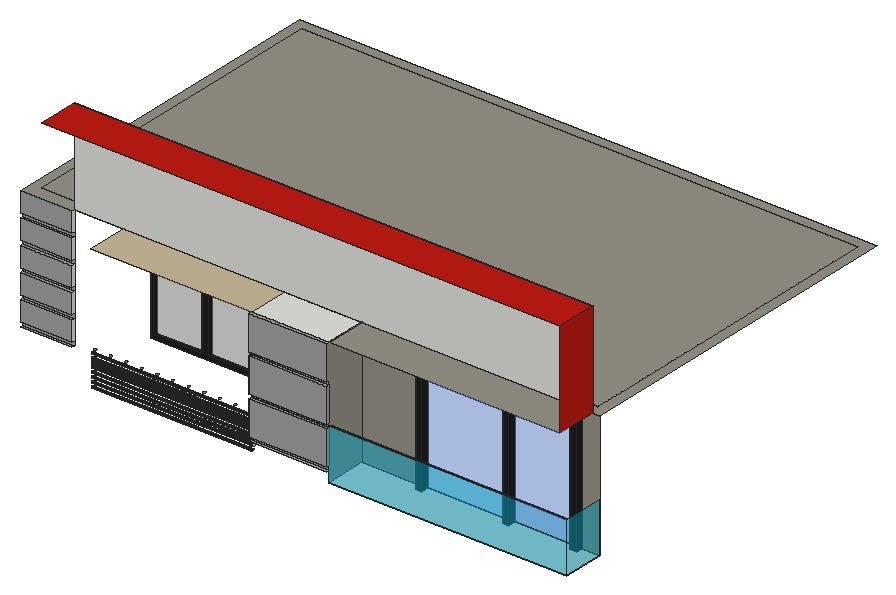
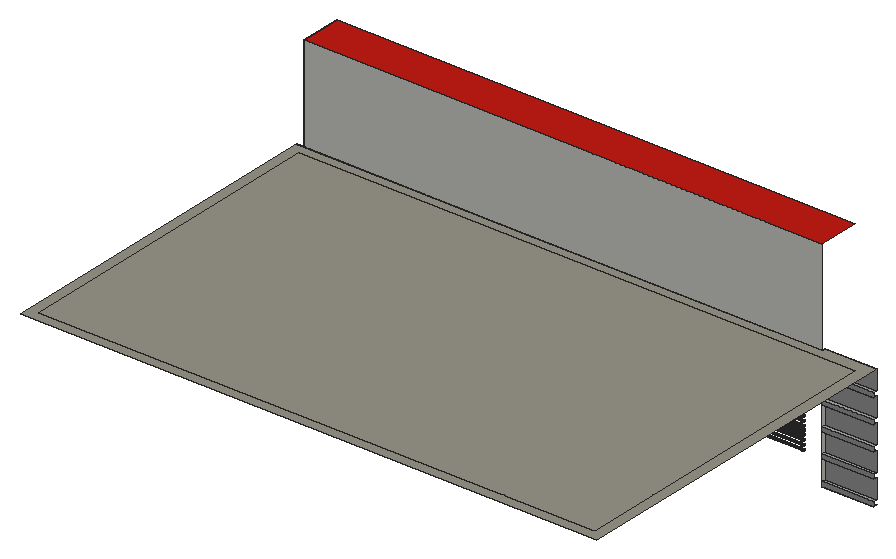
# SketchUp Ruby script. Lengths in inches.
U = 1.inch
M = Sketchup.active_model
def pt(a) = Geom::Point3d.new(a.map { |v| v * U })
def face(e, loops, mat)
  f = e.add_face(loops[0].map { |a| pt(a) })
  loops[1..].each { |l| e.add_face(l.map { |a| pt(a) }).erase! }
  f.material = f.back_material = mat if mat
  f
end
# faces: each face lists its corners as indices into pts; further lists are holes
def faces(e, pts, list, mat = nil) = list.each { |f| face(e, (f[0].is_a?(Array) ? f : [f]).map { |l| l.map { |i| pts[i] } }, mat) }
# xy, xz, yz: faces in a plane at the given z, y or x. An outline is a flat list of corners, or four numbers for a rectangle; further outlines are holes
def ring(l) = l.size == 4 ? [[l[0], l[1]], [l[2], l[1]], [l[2], l[3]], [l[0], l[3]]] : l.each_slice(2).to_a
def flat(e, list, mat, &to3) = list.each { |f| face(e, (f[0].is_a?(Array) ? f : [f]).map { |l| ring(l).map { |u, v| to3.(u, v) } }, mat) }
def xy(e, z, list, mat = nil) = flat(e, list, mat) { |x, y| [x, y, z] }
def xz(e, y, list, mat = nil) = flat(e, list, mat) { |x, z| [x, y, z] }
def yz(e, x, list, mat = nil) = flat(e, list, mat) { |y, z| [x, y, z] }
def lines(e, pts, list) = list.each { |a, b| e.add_line(pt(pts[a]), pt(pts[b])) }
# prism: a flat outline (further loops are holes) pulled along v
def prism(e, loops, v, mat = nil)
  f = face(e, loops, mat); d = Geom::Vector3d.new(v.map { |x| x * U })
  f.pushpull(f.normal.samedirection?(d) ? d.length : -d.length)
end
def box(e, o, s, mat = nil) = prism(e, [[o, [o[0] + s[0], o[1], o[2]], [o[0] + s[0], o[1] + s[1], o[2]], [o[0], o[1] + s[1], o[2]]]], [0, 0, s[2]], mat)
def at(x, y, z, deg = 0) = Geom::Transformation.translation(pt([x, y, z])) * Geom::Transformation.rotation(ORIGIN, Z_AXIS, deg.degrees)
def axes(o, x, y, z) = Geom::Transformation.new([*x, 0, *y, 0, *z, 0, *pt(o).to_a, 1])
def part(name) = M.definitions.add(name)
# library, detail: a bought-in or finely detailed component or shape, given as its bounding box
def library(name, o, s) = part(name).tap { |d| box(d.entities, o, s) }
def detail(e, o, s) = box(e.add_group.entities, o, s)
def put(e, d, t, mat = nil) = e.add_instance(d, t).tap { |i| i.material = mat if mat }
def group(e, t, mat = nil) = e.add_group.tap { |g| g.transformation = t; g.material = mat if mat }.entities
root = M.entities
M.materials.add("[0133_Gray]").color = [128, 128, 128]
M.materials.add("[Blacktop New]").color = [30, 30, 30]
M.materials.add("[Formica Graystone]").color = [149, 146, 135]
M.materials.add("[Marble Carrara Gold Floor Tile]").color = [225, 223, 217]
M.materials.add("[Modern Siding]").color = [191, 28, 19]
M.materials.add("[Pavers Flagstone Gray]").color = [162, 162, 162]
M.materials.add("[Quartz Light Brown]").color = [199, 184, 152]
M.materials.add("[Translucent Glass Blue]").color = [100, 149, 237]
M.materials["[Translucent Glass Blue]"].alpha = 0.5
M.materials.add("[Translucent Glass Gray]").color = [128, 128, 128]
M.materials["[Translucent Glass Gray]"].alpha = 0.5
M.materials.add("[Translucent Glass Tinted]").color = [8, 201, 241]
M.materials["[Translucent Glass Tinted]"].alpha = 0.48
xy(root,489.7,[[349.36,33,355.36,39],[425.89,33,431.59,39],[484.98,33,490.98,39]])
xy(root,489.7,[[297.58,3,506.625,3,506.625,39,490.98,39,490.98,33,484.98,33,484.98,39,431.59,39,431.59,33,425.89,33,425.89,39,355.36,39,355.36,33,349.36,33,349.36,39,297.58,39]],"[Marble Carrara Gold Floor Tile]")
xy(root,492.8125,[[0,36,45.0625,39]],"[Pavers Flagstone Gray]")
xy(root,496.89,[[0,36,45.0625,39]],"[Pavers Flagstone Gray]")
xy(root,499.5,[[229.62,0,297.58,3]],"[Pavers Flagstone Gray]")
xy(root,503.12,[[229.62,0,297.58,3]],"[Pavers Flagstone Gray]")
xy(root,514.25,[[0,36,45.0625,39]],"[Pavers Flagstone Gray]")
xy(root,518.32,[[0,36,45.0625,39]],"[Pavers Flagstone Gray]")
xy(root,521.04,[[91.04,3.35,91.27,3.36,91.48,3.43,91.68,3.55,91.83,3.73,91.93,3.93,91.98,4.15,91.96,4.38,91.89,4.6,91.77,4.79,91.6,4.94,91.39,5.04,91.17,5.09,90.94,5.08,90.72,5.01,90.53,4.88,90.38,4.71,90.28,4.51,90.23,4.28,90.24,4.05,90.32,3.84,90.44,3.65,90.61,3.49,90.82,3.39],[104.73,3.35,104.95,3.36,105.17,3.43,105.36,3.55,105.51,3.73,105.62,3.93,105.66,4.15,105.65,4.38,105.58,4.6,105.45,4.79,105.28,4.94,105.08,5.04,104.86,5.09,104.63,5.08,104.41,5.01,104.22,4.88,104.07,4.71,103.97,4.51,103.92,4.28,103.93,4.05,104,3.84,104.13,3.65,104.3,3.49,104.5,3.39],[118.41,3.35,118.64,3.36,118.86,3.43,119.05,3.55,119.2,3.73,119.31,3.93,119.35,4.15,119.34,4.38,119.27,4.6,119.14,4.79,118.97,4.94,118.77,5.04,118.54,5.09,118.32,5.08,118.1,5.01,117.91,4.88,117.76,4.71,117.65,4.51,117.61,4.28,117.62,4.05,117.69,3.84,117.82,3.65,117.99,3.49,118.19,3.39],[132.1,3.35,132.33,3.36,132.55,3.43,132.74,3.55,132.89,3.73,132.99,3.93,133.04,4.15,133.03,4.38,132.95,4.6,132.83,4.79,132.66,4.94,132.46,5.04,132.23,5.09,132,5.08,131.79,5.01,131.6,4.88,131.44,4.71,131.34,4.51,131.29,4.28,131.31,4.05,131.38,3.84,131.5,3.65,131.67,3.49,131.88,3.39],[145.79,3.35,146.02,3.36,146.23,3.43,146.43,3.55,146.58,3.73,146.68,3.93,146.73,4.15,146.71,4.38,146.64,4.6,146.52,4.79,146.35,4.94,146.14,5.04,145.92,5.09,145.69,5.08,145.47,5.01,145.28,4.88,145.13,4.71,145.03,4.51,144.98,4.28,144.99,4.05,145.07,3.84,145.19,3.65,145.36,3.49,145.57,3.39],
  [159.48,3.35,159.7,3.36,159.92,3.43,160.11,3.55,160.26,3.73,160.37,3.93,160.41,4.15,160.4,4.38,160.33,4.6,160.2,4.79,160.03,4.94,159.83,5.04,159.61,5.09,159.38,5.08,159.16,5.01,158.97,4.88,158.82,4.71,158.72,4.51,158.67,4.28,158.68,4.05,158.75,3.84,158.88,3.65,159.05,3.49,159.25,3.39],[173.16,3.35,173.39,3.36,173.61,3.43,173.8,3.55,173.95,3.73,174.06,3.93,174.1,4.15,174.09,4.38,174.02,4.6,173.89,4.79,173.72,4.94,173.52,5.04,173.29,5.09,173.07,5.08,172.85,5.01,172.66,4.88,172.51,4.71,172.4,4.51,172.36,4.28,172.37,4.05,172.44,3.84,172.57,3.65,172.74,3.49,172.94,3.39],[186.85,3.35,187.08,3.36,187.3,3.43,187.49,3.55,187.64,3.73,187.74,3.93,187.79,4.15,187.78,4.38,187.7,4.6,187.58,4.79,187.41,4.94,187.21,5.04,186.98,5.09,186.75,5.08,186.54,5.01,186.35,4.88,186.19,4.71,186.09,4.51,186.04,4.28,186.06,4.05,186.13,3.84,186.25,3.65,186.42,3.49,186.63,3.39],[200.54,3.35,200.77,3.36,200.98,3.43,201.18,3.55,201.33,3.73,201.43,3.93,201.48,4.15,201.46,4.38,201.39,4.6,201.27,4.79,201.1,4.94,200.89,5.04,200.67,5.09,200.44,5.08,200.22,5.01,200.03,4.88,199.88,4.71,199.78,4.51,199.73,4.28,199.74,4.05,199.82,3.84,199.94,3.65,200.11,3.49,200.32,3.39],[214.23,3.35,214.45,3.36,214.67,3.43,214.86,3.55,215.01,3.73,215.12,3.93,215.16,4.15,215.15,4.38,215.08,4.6,214.95,4.79,214.78,4.94,214.58,5.04,214.36,5.09,214.13,5.08,213.91,5.01,213.72,4.88,213.57,4.71,213.47,4.51,213.42,4.28,213.43,4.05,213.5,3.84,213.63,3.65,213.8,3.49,214,3.39],
  [227.91,3.35,228.14,3.36,228.36,3.43,228.55,3.55,228.7,3.73,228.81,3.93,228.85,4.15,228.84,4.38,228.77,4.6,228.64,4.79,228.47,4.94,228.27,5.04,228.04,5.09,227.82,5.08,227.6,5.01,227.41,4.88,227.26,4.71,227.15,4.51,227.11,4.28,227.12,4.05,227.19,3.84,227.32,3.65,227.49,3.49,227.69,3.39]],"[0133_Gray]")
xy(root,524.95,[[114.78,36,204.16,39]])
xy(root,527.95,[[117.78,36,159.47,39],[165.58,36,201.16,39]],"[Blacktop New]")
xy(root,533,[[229.62,0,297.58,3]],"[Pavers Flagstone Gray]")
xy(root,534.06,[[297.58,3,506.625,3.25]])
xy(root,534.56,[[297.58,3,506.625,3.25]])
xy(root,535.6875,[[0,36,45.0625,39]],"[Pavers Flagstone Gray]")
xy(root,536.62,[[229.62,0,297.58,3]],"[Pavers Flagstone Gray]")
xy(root,539.76,[[0,36,45.0625,39]],"[Pavers Flagstone Gray]")
xy(root,557.125,[[0,36,45.0625,39]],"[Pavers Flagstone Gray]")
xy(root,561.2,[[0,36,45.0625,39]],"[Pavers Flagstone Gray]")
xy(root,566.5,[[229.62,0,297.58,3]],"[Pavers Flagstone Gray]")
xy(root,570.12,[[229.62,0,297.58,3]],"[Pavers Flagstone Gray]")
xy(root,578.5625,[[0,36,45.0625,39]],"[Pavers Flagstone Gray]")
xy(root,582.64,[[0,36,45.0625,39]],"[Pavers Flagstone Gray]")
xy(root,587.51,[[355.36,33,425.89,39],[431.59,33,484.98,39]],"[Blacktop New]")
xy(root,590.82,[[117.78,36,159.47,39],[165.58,36,201.16,39]],"[Blacktop New]")
xy(root,593.51,[[349.36,33,490.98,39]],"[Blacktop New]")
xy(root,593.82,[[114.78,36,204.16,39]],"[Blacktop New]")
xy(root,600,[[229.62,3,297.58,39]])
xy(root,600,[[297.58,3,500.56,39],[[0,36,45.0625,36,45.0625,39,506.625,39,506.625,342.4375,0,342.4375],[9,48,497.625,333.4375]],[9,48,497.625,333.4375]],"[Formica Graystone]")
xy(root,600,[[229.62,0,297.58,3]],"[Pavers Flagstone Gray]")
xy(root,600,[[88.53,3,229.62,39]],"[Quartz Light Brown]")
xy(root,683.96,[[45.0625,3,500.56,39]],"[Modern Siding]")
xz(root,0,[[229.62,503.12,297.58,533],[229.62,536.62,297.58,566.5],[229.62,570.12,297.58,600]],"[Pavers Flagstone Gray]")
xz(root,3,[[229.62,503.12,297.58,533],[229.62,536.62,297.58,566.5]])
xz(root,3,[[229.62,499.5,297.58,503.12],[229.62,533,297.58,533,297.58,534.06,506.625,534.06,506.625,534.56,297.58,534.56,297.58,536.62,229.62,536.62],[229.62,566.5,297.58,570.12]],"[Pavers Flagstone Gray]")
xz(root,3,[[297.58,489.7,506.625,534.06]],"[Translucent Glass Tinted]")
xz(root,3.25,[[297.58,534.06,506.625,534.56]])
xz(root,33,[[349.36,489.7,355.36,489.7,355.36,587.51,425.89,587.51,425.89,489.7,431.59,489.7,431.59,587.51,484.98,587.51,484.98,489.7,490.98,489.7,490.98,593.51,349.36,593.51]],"[Blacktop New]")
xz(root,36,[[[114.78,524.95,204.16,593.82],[117.78,527.95,159.47,590.82],[165.58,527.95,201.16,590.82]]],"[Blacktop New]")
xz(root,36,[[0,496.89,45.0625,514.25],[0,518.32,45.0625,535.6875],[0,539.76,45.0625,557.125],[0,561.2,45.0625,578.5625],[0,582.64,45.0625,600]],"[Pavers Flagstone Gray]")
xz(root,39,[[425.89,489.7,431.59,587.51],[45.0625,600,500.56,683.96]])
xz(root,39,[[297.58,489.7,349.36,489.7,349.36,593.51,490.98,593.51,490.98,489.7,506.625,489.7,506.625,600,297.58,600]],"[Formica Graystone]")
xz(root,39,[[0,492.8125,45.0625,496.89],[0,514.25,45.0625,518.32],[0,535.6875,45.0625,539.76],[0,557.125,45.0625,561.2],[0,578.5625,45.0625,582.64]],"[Pavers Flagstone Gray]")
xz(root,39,[[355.36,489.7,425.89,587.51],[431.59,489.7,484.98,587.51]],"[Translucent Glass Blue]")
xz(root,39,[[117.78,527.95,159.47,590.82],[165.58,527.95,201.16,590.82]],"[Translucent Glass Gray]")
yz(root,45.0625,[[36,496.89,39,514.25],[36,518.32,39,535.6875],[36,539.76,39,557.125],[36,561.2,39,578.5625],[36,582.64,39,600]])
yz(root,114.78,[[36,524.95,39,593.82]],"[Blacktop New]")
yz(root,117.78,[[36,527.95,39,590.82]],"[Blacktop New]")
yz(root,159.47,[[36,527.95,39,590.82]],"[Blacktop New]")
yz(root,165.58,[[36,527.95,39,590.82]],"[Blacktop New]")
yz(root,201.16,[[36,527.95,39,590.82]],"[Blacktop New]")
yz(root,204.16,[[36,524.95,39,593.82]],"[Blacktop New]")
yz(root,229.62,[[0,503.12,3,533],[0,536.62,3,566.5]],"[Pavers Flagstone Gray]")
yz(root,230.47,[[4.3,494.1,4.51,494.13,4.71,494.21,4.88,494.34,5.01,494.51,5.09,494.71,5.12,494.92,5.09,495.125,5.01,495.32,4.88,495.49,4.71,495.62,4.51,495.7,4.3,495.73,4.09,495.7,3.9,495.62,3.73,495.49,3.6,495.32,3.52,495.125,3.49,494.92,3.52,494.71,3.6,494.51,3.73,494.34,3.9,494.21,4.09,494.13]])
yz(root,230.66,[[4.3,497.92,4.51,497.94,4.71,498.02,4.88,498.15,5.01,498.32,5.09,498.52,5.12,498.73,5.09,498.9375,5.01,499.13,4.88,499.3,4.71,499.43,4.51,499.51,4.3,499.54,4.09,499.51,3.9,499.43,3.73,499.3,3.6,499.13,3.52,498.9375,3.49,498.73,3.52,498.52,3.6,498.32,3.73,498.15,3.9,498.02,4.09,497.94]])
yz(root,297.58,[[3,489.7,39,489.7,39,600,0,600,0,570.12,3,570.12,3,534.56,3.25,534.56,3.25,534.06,3,534.06]],"[Formica Graystone]")
yz(root,297.58,[[0,503.12,3,533],[0,536.62,3,566.5]],"[Pavers Flagstone Gray]")
yz(root,349.36,[[33,489.7,39,593.51]],"[Blacktop New]")
yz(root,355.36,[[33,489.7,39,587.51]],"[Blacktop New]")
yz(root,425.89,[[33,489.7,39,587.51]],"[Blacktop New]")
yz(root,431.59,[[33,489.7,39,587.51]],"[Blacktop New]")
yz(root,484.98,[[33,489.7,39,587.51]],"[Blacktop New]")
yz(root,490.98,[[33,489.7,39,593.51]],"[Blacktop New]")
yz(root,500.56,[[3,600,39,683.96]],"[Modern Siding]")
yz(root,506.625,[[3,534.06,3.25,534.56]])
yz(root,506.625,[[3,489.7,39,533.64]],"[Translucent Glass Tinted]")
p = [[88.53,3.9,490.4],[88.53,4.09,490.32],[229.62,4.09,490.32],[229.62,3.9,490.4],[88.53,4.3,490.29],[229.62,4.3,490.29],
  [88.53,4.51,490.32],[229.62,4.51,490.32],[88.53,4.71,490.4],[229.62,4.71,490.4],[88.53,3.73,490.53],[229.62,3.73,490.53],
  [88.53,4.88,490.53],[229.62,4.88,490.53],[88.53,3.6,490.7],[229.62,3.6,490.7],[88.53,5.01,490.7],[90.72,5.01,490.7],
  [104.41,5.01,490.7],[118.1,5.01,490.7],[131.79,5.01,490.7],[145.47,5.01,490.7],[159.16,5.01,490.7],[172.85,5.01,490.7],
  [186.54,5.01,490.7],[200.22,5.01,490.7],[213.91,5.01,490.7],[227.6,5.01,490.7],[229.62,5.01,490.7],[88.53,3.52,490.89],
  [229.62,3.52,490.89],[88.53,5.09,490.89],[229.62,5.09,490.89],[88.53,3.49,491.1],[229.62,3.49,491.1],[88.53,5.12,491.1],
  [229.62,5.12,491.1],[88.53,3.52,491.3125],[229.62,3.52,491.3125],[88.53,5.09,491.3125],[229.62,5.09,491.3125],[88.53,3.6,491.51],
  [229.62,3.6,491.51],[88.53,5.01,491.51],[90.72,5.01,491.51],[104.41,5.01,491.51],[118.1,5.01,491.51],[131.79,5.01,491.51],
  [145.47,5.01,491.51],[159.16,5.01,491.51],[172.85,5.01,491.51],[186.54,5.01,491.51],[200.22,5.01,491.51],[213.91,5.01,491.51],
  [227.6,5.01,491.51],[229.62,5.01,491.51],[88.53,3.73,491.68],[229.62,3.73,491.68],[88.53,4.88,491.68],[229.62,4.88,491.68],
  [88.53,3.9,491.81],[229.62,3.9,491.81],[88.53,4.71,491.81],[229.62,4.71,491.81],[88.53,4.09,491.89],[229.62,4.09,491.89],
  [88.53,4.51,491.89],[229.62,4.51,491.89],[88.53,4.3,491.92],[229.62,4.3,491.92],[88.53,3.9,494.21],[88.53,4.09,494.13],
  [230.47,4.09,494.13],[230.47,3.9,494.21],[88.53,4.3,494.1],[230.47,4.3,494.1],[88.53,4.51,494.13],[230.47,4.51,494.13],
  [88.53,4.71,494.21],[230.47,4.71,494.21],[88.53,3.73,494.34],[230.47,3.73,494.34],[88.53,4.88,494.34],[230.47,4.88,494.34],
  [88.53,3.6,494.51],[230.47,3.6,494.51],[88.53,5.01,494.51],[90.72,5.01,494.51],[104.41,5.01,494.51],[118.1,5.01,494.51],
  [131.79,5.01,494.51],[145.47,5.01,494.51],[159.16,5.01,494.51],[172.85,5.01,494.51],[186.54,5.01,494.51],[200.22,5.01,494.51],
  [213.91,5.01,494.51],[227.6,5.01,494.51],[230.47,5.01,494.51],[88.53,3.52,494.71],[230.47,3.52,494.71],[88.53,5.09,494.71],
  [230.47,5.09,494.71],[88.53,3.49,494.92],[230.47,3.49,494.92],[88.53,5.12,494.92],[230.47,5.12,494.92],[88.53,3.52,495.125],
  [230.47,3.52,495.125],[88.53,5.09,495.125],[230.47,5.09,495.125],[88.53,3.6,495.32],[230.47,3.6,495.32],[88.53,5.01,495.32],
  [90.72,5.01,495.32],[104.41,5.01,495.32],[118.1,5.01,495.32],[131.79,5.01,495.32],[145.47,5.01,495.32],[159.16,5.01,495.32],
  [172.85,5.01,495.32],[186.54,5.01,495.32],[200.22,5.01,495.32],[213.91,5.01,495.32],[227.6,5.01,495.32],[230.47,5.01,495.32],
  [88.53,3.73,495.49],[230.47,3.73,495.49],[88.53,4.88,495.49],[230.47,4.88,495.49],[88.53,3.9,495.62],[230.47,3.9,495.62],
  [88.53,4.71,495.62],[230.47,4.71,495.62],[88.53,4.09,495.7],[230.47,4.09,495.7],[88.53,4.51,495.7],[230.47,4.51,495.7],
  [88.53,4.3,495.73],[230.47,4.3,495.73],[88.53,3.9,498.02],[88.53,4.09,497.94],[230.66,4.09,497.94],[230.66,3.9,498.02],
  [88.53,4.3,497.92],[230.66,4.3,497.92],[88.53,4.51,497.94],[230.66,4.51,497.94],[88.53,4.71,498.02],[230.66,4.71,498.02],
  [88.53,3.73,498.15],[230.66,3.73,498.15],[88.53,4.88,498.15],[230.66,4.88,498.15],[88.53,3.6,498.32],[230.66,3.6,498.32],
  [88.53,5.01,498.32],[90.72,5.01,498.32],[104.41,5.01,498.32],[118.1,5.01,498.32],[131.79,5.01,498.32],[145.47,5.01,498.32],
  [159.16,5.01,498.32],[172.85,5.01,498.32],[186.54,5.01,498.32],[200.22,5.01,498.32],[213.91,5.01,498.32],[227.6,5.01,498.32],
  [230.66,5.01,498.32],[88.53,3.52,498.52],[230.66,3.52,498.52],[88.53,5.09,498.52],[230.66,5.09,498.52],[88.53,3.49,498.73],
  [230.66,3.49,498.73],[88.53,5.12,498.73],[230.66,5.12,498.73],[88.53,3.52,498.9375],[230.66,3.52,498.9375],[88.53,5.09,498.9375],
  [230.66,5.09,498.9375],[88.53,3.6,499.13],[230.66,3.6,499.13],[88.53,5.01,499.13],[90.72,5.01,499.13],[104.41,5.01,499.13],
  [118.1,5.01,499.13],[131.79,5.01,499.13],[145.47,5.01,499.13],[159.16,5.01,499.13],[172.85,5.01,499.13],[186.54,5.01,499.13],
  [200.22,5.01,499.13],[213.91,5.01,499.13],[227.6,5.01,499.13],[230.66,5.01,499.13],[88.53,3.73,499.3],[230.66,3.73,499.3],
  [88.53,4.88,499.3],[230.66,4.88,499.3],[88.53,3.9,499.43],[230.66,3.9,499.43],[88.53,4.71,499.43],[230.66,4.71,499.43],
  [88.53,4.09,499.51],[230.66,4.09,499.51],[88.53,4.51,499.51],[230.66,4.51,499.51],[88.53,4.3,499.54],[230.66,4.3,499.54],
  [88.53,4.09,501.76],[88.53,4.3,501.73],[229.62,4.3,501.73],[229.62,4.09,501.76],[88.53,4.51,501.76],[229.62,4.51,501.76],
  [88.53,3.73,501.97],[88.53,3.9,501.84],[229.62,3.9,501.84],[229.62,3.73,501.97],[88.53,4.71,501.84],[229.62,4.71,501.84],
  [88.53,4.88,501.97],[229.62,4.88,501.97],[88.53,3.6,502.13],[229.62,3.6,502.13],[88.53,5.01,502.13],[90.72,5.01,502.13],
  [104.41,5.01,502.13],[118.1,5.01,502.13],[131.79,5.01,502.13],[145.47,5.01,502.13],[159.16,5.01,502.13],[172.85,5.01,502.13],
  [186.54,5.01,502.13],[200.22,5.01,502.13],[213.91,5.01,502.13],[227.6,5.01,502.13],[229.62,5.01,502.13],[88.53,3.52,502.33],
  [229.62,3.52,502.33],[88.53,5.09,502.33],[229.62,5.09,502.33],[88.53,3.49,502.54],[229.62,3.49,502.54],[88.53,5.12,502.54],
  [229.62,5.12,502.54],[88.53,3.52,502.75],[229.62,3.52,502.75],[88.53,5.09,502.75],[229.62,5.09,502.75],[88.53,3.6,502.95],
  [229.62,3.6,502.95],[88.53,5.01,502.95],[90.72,5.01,502.95],[104.41,5.01,502.95],[118.1,5.01,502.95],[131.79,5.01,502.95],
  [145.47,5.01,502.95],[159.16,5.01,502.95],[172.85,5.01,502.95],[186.54,5.01,502.95],[200.22,5.01,502.95],[213.91,5.01,502.95],
  [227.6,5.01,502.95],[229.62,5.01,502.95],[88.53,3.73,503.11],[229.62,3.73,503.11],[88.53,4.88,503.11],[229.62,4.88,503.11],
  [88.53,3.9,503.24],[229.62,3.9,503.24],[88.53,4.71,503.24],[229.62,4.71,503.24],[88.53,4.09,503.33],[229.62,4.09,503.33],
  [88.53,4.51,503.33],[229.62,4.51,503.33],[88.53,4.3,503.35],[229.62,4.3,503.35],[88.53,4.09,505.57],[88.53,4.3,505.54],
  [229.62,4.3,505.54],[229.62,4.09,505.57],[88.53,4.51,505.57],[229.62,4.51,505.57],[88.53,3.73,505.78],[88.53,3.9,505.65],
  [229.62,3.9,505.65],[229.62,3.73,505.78],[88.53,4.71,505.65],[229.62,4.71,505.65],[88.53,4.88,505.78],[229.62,4.88,505.78],
  [88.53,3.6,505.95],[229.62,3.6,505.95],[88.53,5.01,505.95],[90.72,5.01,505.95],[104.41,5.01,505.95],[118.1,5.01,505.95],
  [131.79,5.01,505.95],[145.47,5.01,505.95],[159.16,5.01,505.95],[172.85,5.01,505.95],[186.54,5.01,505.95],[200.22,5.01,505.95],
  [213.91,5.01,505.95],[227.6,5.01,505.95],[229.62,5.01,505.95],[88.53,3.52,506.14],[229.62,3.52,506.14],[88.53,5.09,506.14],
  [229.62,5.09,506.14],[88.53,3.49,506.35],[229.62,3.49,506.35],[88.53,5.12,506.35],[229.62,5.12,506.35],[88.53,3.52,506.5625],
  [229.62,3.52,506.5625],[88.53,5.09,506.5625],[229.62,5.09,506.5625],[88.53,3.6,506.76],[229.62,3.6,506.76],[88.53,5.01,506.76],
  [90.72,5.01,506.76],[104.41,5.01,506.76],[118.1,5.01,506.76],[131.79,5.01,506.76],[145.47,5.01,506.76],[159.16,5.01,506.76],
  [172.85,5.01,506.76],[186.54,5.01,506.76],[200.22,5.01,506.76],[213.91,5.01,506.76],[227.6,5.01,506.76],[229.62,5.01,506.76],
  [88.53,3.73,506.93],[229.62,3.73,506.93],[88.53,4.88,506.93],[229.62,4.88,506.93],[88.53,3.9,507.06],[229.62,3.9,507.06],
  [88.53,4.71,507.06],[229.62,4.71,507.06],[88.53,4.09,507.14],[229.62,4.09,507.14],[88.53,4.3,507.17],[229.62,4.3,507.17],
  [88.53,4.51,507.14],[229.62,4.51,507.14],[88.53,3.9,509.46],[88.53,4.09,509.38],[229.62,4.09,509.38],[229.62,3.9,509.46],
  [88.53,4.3,509.35],[229.62,4.3,509.35],[88.53,4.51,509.38],[229.62,4.51,509.38],[88.53,4.71,509.46],[229.62,4.71,509.46],
  [88.53,3.73,509.59],[229.62,3.73,509.59],[88.53,4.88,509.59],[229.62,4.88,509.59],[88.53,3.6,509.76],[229.62,3.6,509.76],
  [88.53,5.01,509.76],[90.72,5.01,509.76],[104.41,5.01,509.76],[118.1,5.01,509.76],[131.79,5.01,509.76],[145.47,5.01,509.76],
  [159.16,5.01,509.76],[172.85,5.01,509.76],[186.54,5.01,509.76],[200.22,5.01,509.76],[213.91,5.01,509.76],[227.6,5.01,509.76],
  [229.62,5.01,509.76],[88.53,3.52,509.96],[229.62,3.52,509.96],[88.53,5.09,509.96],[229.62,5.09,509.96],[88.53,3.49,510.17],
  [229.62,3.49,510.17],[88.53,5.12,510.17],[229.62,5.12,510.17],[88.53,3.52,510.375],[229.62,3.52,510.375],[88.53,5.09,510.375],
  [229.62,5.09,510.375],[88.53,3.6,510.57],[229.62,3.6,510.57],[88.53,5.01,510.57],[90.72,5.01,510.57],[104.41,5.01,510.57],
  [118.1,5.01,510.57],[131.79,5.01,510.57],[145.47,5.01,510.57],[159.16,5.01,510.57],[172.85,5.01,510.57],[186.54,5.01,510.57],
  [200.22,5.01,510.57],[213.91,5.01,510.57],[227.6,5.01,510.57],[229.62,5.01,510.57],[88.53,3.73,510.74],[229.62,3.73,510.74],
  [88.53,4.88,510.74],[229.62,4.88,510.74],[88.53,3.9,510.87],[229.62,3.9,510.87],[88.53,4.71,510.87],[229.62,4.71,510.87],
  [88.53,4.09,510.95],[229.62,4.09,510.95],[88.53,4.51,510.95],[229.62,4.51,510.95],[88.53,4.3,510.98],[229.62,4.3,510.98],
  [88.53,3.9,513.27],[88.53,4.09,513.19],[229.62,4.09,513.19],[229.62,3.9,513.27],[88.53,4.3,513.17],[229.62,4.3,513.17],
  [88.53,4.51,513.19],[229.62,4.51,513.19],[88.53,4.71,513.27],[229.62,4.71,513.27],[88.53,3.73,513.4],[229.62,3.73,513.4],
  [88.53,4.88,513.4],[229.62,4.88,513.4],[88.53,3.6,513.57],[229.62,3.6,513.57],[88.53,5.01,513.57],[90.72,5.01,513.57],
  [104.41,5.01,513.57],[118.1,5.01,513.57],[131.79,5.01,513.57],[145.47,5.01,513.57],[159.16,5.01,513.57],[172.85,5.01,513.57],
  [186.54,5.01,513.57],[200.22,5.01,513.57],[213.91,5.01,513.57],[227.6,5.01,513.57],[229.62,5.01,513.57],[88.53,3.52,513.77],
  [229.62,3.52,513.77],[88.53,5.09,513.77],[229.62,5.09,513.77],[88.53,3.49,513.98],[229.62,3.49,513.98],[88.53,5.12,513.98],
  [229.62,5.12,513.98],[88.53,3.52,514.1875],[229.62,3.52,514.1875],[88.53,5.09,514.1875],[229.62,5.09,514.1875],[88.53,3.6,514.38],
  [229.62,3.6,514.38],[88.53,5.01,514.38],[90.72,5.01,514.38],[104.41,5.01,514.38],[118.1,5.01,514.38],[131.79,5.01,514.38],
  [145.47,5.01,514.38],[159.16,5.01,514.38],[172.85,5.01,514.38],[186.54,5.01,514.38],[200.22,5.01,514.38],[213.91,5.01,514.38],
  [227.6,5.01,514.38],[229.62,5.01,514.38],[88.53,3.73,514.55],[229.62,3.73,514.55],[88.53,4.88,514.55],[229.62,4.88,514.55],
  [88.53,3.9,514.68],[229.62,3.9,514.68],[88.53,4.71,514.68],[229.62,4.71,514.68],[88.53,4.09,514.76],[229.62,4.09,514.76],
  [88.53,4.51,514.76],[229.62,4.51,514.76],[88.53,4.3,514.79],[229.62,4.3,514.79],[88.53,3.9,517.09],[88.53,4.09,517.01],
  [229.62,4.09,517.01],[229.62,3.9,517.09],[88.53,4.3,516.98],[229.62,4.3,516.98],[88.53,4.51,517.01],[229.62,4.51,517.01],
  [88.53,4.71,517.09],[229.62,4.71,517.09],[88.53,3.73,517.22],[229.62,3.73,517.22],[88.53,4.88,517.22],[229.62,4.88,517.22],
  [88.53,3.6,517.38],[229.62,3.6,517.38],[88.53,5.01,517.38],[90.72,5.01,517.38],[104.41,5.01,517.38],[118.1,5.01,517.38],
  [131.79,5.01,517.38],[145.47,5.01,517.38],[159.16,5.01,517.38],[172.85,5.01,517.38],[186.54,5.01,517.38],[200.22,5.01,517.38],
  [213.91,5.01,517.38],[227.6,5.01,517.38],[229.62,5.01,517.38],[88.53,3.52,517.58],[229.62,3.52,517.58],[88.53,5.09,517.58],
  [229.62,5.09,517.58],[88.53,3.49,517.79],[229.62,3.49,517.79],[88.53,5.12,517.79],[229.62,5.12,517.79],[88.53,3.52,518],
  [229.62,3.52,518],[88.53,5.09,518],[229.62,5.09,518],[88.53,3.6,518.2],[229.62,3.6,518.2],[88.53,5.01,518.2],
  [90.72,5.01,518.2],[104.41,5.01,518.2],[118.1,5.01,518.2],[131.79,5.01,518.2],[145.47,5.01,518.2],[159.16,5.01,518.2],
  [172.85,5.01,518.2],[186.54,5.01,518.2],[200.22,5.01,518.2],[213.91,5.01,518.2],[227.6,5.01,518.2],[229.62,5.01,518.2],
  [88.53,3.73,518.36],[229.62,3.73,518.36],[88.53,4.88,518.36],[229.62,4.88,518.36],[88.53,3.9,518.49],[229.62,3.9,518.49],
  [88.53,4.71,518.49],[229.62,4.71,518.49],[88.53,4.09,518.58],[229.62,4.09,518.58],[88.53,4.51,518.58],[229.62,4.51,518.58],
  [88.53,4.3,518.6],[229.62,4.3,518.6]]
faces(root,p,[[0,1,2,3],[1,4,5,2],[4,6,7,5],[6,8,9,7],[10,0,3,11],[8,12,13,9],[14,10,11,15],[12,16,17,18,19,20,21,22,23,24,25,26,27,28,13],
  [29,14,15,30],[16,31,32,28,27,26,25,24,23,22,21,20,19,18,17],[33,29,30,34],[31,35,36,32],[37,33,34,38],[35,39,40,36],[41,37,38,42],[39,43,44,45,46,47,48,49,50,51,52,53,54,55,40],
  [56,41,42,57],[43,58,59,55,54,53,52,51,50,49,48,47,46,45,44],[60,56,57,61],[58,62,63,59],[64,60,61,65],[62,66,67,63],[68,64,65,69],[66,68,69,67],
  [70,71,72,73],[71,74,75,72],[74,76,77,75],[76,78,79,77],[80,70,73,81],[78,82,83,79],[84,80,81,85],[82,86,87,88,89,90,91,92,93,94,95,96,97,98,83],
  [99,84,85,100],[86,101,102,98,97,96,95,94,93,92,91,90,89,88,87],[103,99,100,104],[101,105,106,102],[107,103,104,108],[105,109,110,106],[111,107,108,112],[109,113,114,115,116,117,118,119,120,121,122,123,124,125,110],
  [126,111,112,127],[113,128,129,125,124,123,122,121,120,119,118,117,116,115,114],[130,126,127,131],[128,132,133,129],[134,130,131,135],[132,136,137,133],[138,134,135,139],[136,138,139,137],
  [140,141,142,143],[141,144,145,142],[144,146,147,145],[146,148,149,147],[150,140,143,151],[148,152,153,149],[154,150,151,155],[152,156,157,158,159,160,161,162,163,164,165,166,167,168,153],
  [169,154,155,170],[156,171,172,168,167,166,165,164,163,162,161,160,159,158,157],[173,169,170,174],[171,175,176,172],[177,173,174,178],[175,179,180,176],[181,177,178,182],[179,183,184,185,186,187,188,189,190,191,192,193,194,195,180],
  [196,181,182,197],[183,198,199,195,194,193,192,191,190,189,188,187,186,185,184],[200,196,197,201],[198,202,203,199],[204,200,201,205],[202,206,207,203],[208,204,205,209],[206,208,209,207],
  [210,211,212,213],[211,214,215,212],[216,217,218,219],[217,210,213,218],[214,220,221,215],[220,222,223,221],[224,216,219,225],[222,226,227,228,229,230,231,232,233,234,235,236,237,238,223],
  [239,224,225,240],[226,241,242,238,237,236,235,234,233,232,231,230,229,228,227],[243,239,240,244],[241,245,246,242],[247,243,244,248],[245,249,250,246],[251,247,248,252],[249,253,254,255,256,257,258,259,260,261,262,263,264,265,250],
  [266,251,252,267],[253,268,269,265,264,263,262,261,260,259,258,257,256,255,254],[270,266,267,271],[268,272,273,269],[274,270,271,275],[272,276,277,273],[278,274,275,279],[276,278,279,277],
  [280,281,282,283],[281,284,285,282],[286,287,288,289],[287,280,283,288],[284,290,291,285],[290,292,293,291],[294,286,289,295],[292,296,297,298,299,300,301,302,303,304,305,306,307,308,293],
  [309,294,295,310],[296,311,312,308,307,306,305,304,303,302,301,300,299,298,297],[313,309,310,314],[311,315,316,312],[317,313,314,318],[315,319,320,316],[321,317,318,322],[319,323,324,325,326,327,328,329,330,331,332,333,334,335,320],
  [336,321,322,337],[323,338,339,335,334,333,332,331,330,329,328,327,326,325,324],[340,336,337,341],[338,342,343,339],[344,340,341,345],[346,344,345,347],[348,346,347,349],[342,348,349,343],
  [350,351,352,353],[351,354,355,352],[354,356,357,355],[356,358,359,357],[360,350,353,361],[358,362,363,359],[364,360,361,365],[362,366,367,368,369,370,371,372,373,374,375,376,377,378,363],
  [379,364,365,380],[366,381,382,378,377,376,375,374,373,372,371,370,369,368,367],[383,379,380,384],[381,385,386,382],[387,383,384,388],[385,389,390,386],[391,387,388,392],[389,393,394,395,396,397,398,399,400,401,402,403,404,405,390],
  [406,391,392,407],[393,408,409,405,404,403,402,401,400,399,398,397,396,395,394],[410,406,407,411],[408,412,413,409],[414,410,411,415],[412,416,417,413],[418,414,415,419],[416,418,419,417],
  [420,421,422,423],[421,424,425,422],[424,426,427,425],[426,428,429,427],[430,420,423,431],[428,432,433,429],[434,430,431,435],[432,436,437,438,439,440,441,442,443,444,445,446,447,448,433],
  [449,434,435,450],[436,451,452,448,447,446,445,444,443,442,441,440,439,438,437],[453,449,450,454],[451,455,456,452],[457,453,454,458],[455,459,460,456],[461,457,458,462],[459,463,464,465,466,467,468,469,470,471,472,473,474,475,460],
  [476,461,462,477],[463,478,479,475,474,473,472,471,470,469,468,467,466,465,464],[480,476,477,481],[478,482,483,479],[484,480,481,485],[482,486,487,483],[488,484,485,489],[486,488,489,487],
  [490,491,492,493],[491,494,495,492],[494,496,497,495],[496,498,499,497],[500,490,493,501],[498,502,503,499],[504,500,501,505],[502,506,507,508,509,510,511,512,513,514,515,516,517,518,503],
  [519,504,505,520],[506,521,522,518,517,516,515,514,513,512,511,510,509,508,507],[523,519,520,524],[521,525,526,522],[527,523,524,528],[525,529,530,526],[531,527,528,532],[529,533,534,535,536,537,538,539,540,541,542,543,544,545,530],
  [546,531,532,547],[533,548,549,545,544,543,542,541,540,539,538,537,536,535,534],[550,546,547,551],[548,552,553,549],[554,550,551,555],[552,556,557,553],[558,554,555,559],[556,558,559,557]],"[0133_Gray]")
